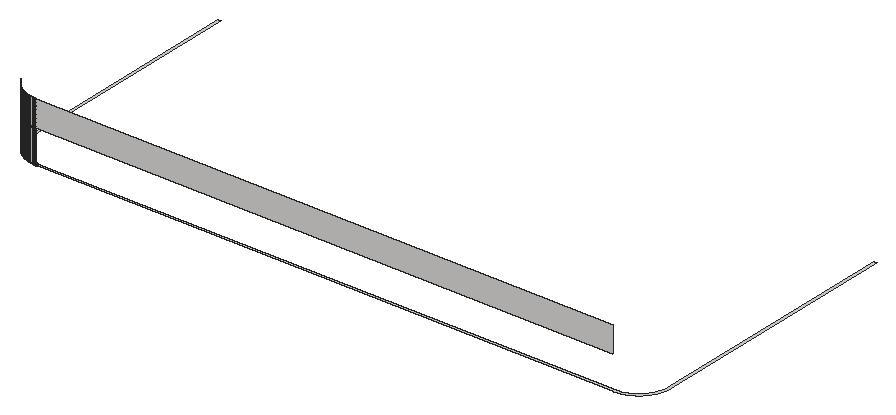
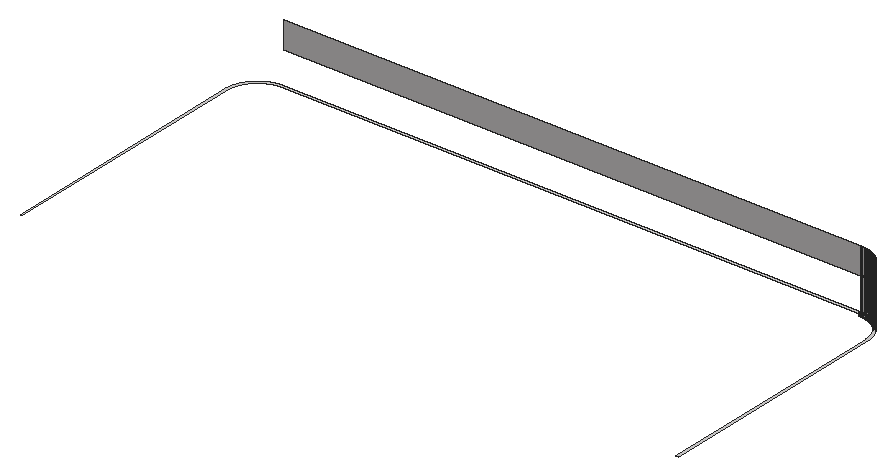
# SketchUp Ruby script. Lengths in inches.
U = 1.inch
M = Sketchup.active_model
def pt(a) = Geom::Point3d.new(a.map { |v| v * U })
def face(e, loops, mat)
  f = e.add_face(loops[0].map { |a| pt(a) })
  loops[1..].each { |l| e.add_face(l.map { |a| pt(a) }).erase! }
  f.material = f.back_material = mat if mat
  f
end
# faces: each face lists its corners as indices into pts; further lists are holes
def faces(e, pts, list, mat = nil) = list.each { |f| face(e, (f[0].is_a?(Array) ? f : [f]).map { |l| l.map { |i| pts[i] } }, mat) }
# xy, xz, yz: faces in a plane at the given z, y or x. An outline is a flat list of corners, or four numbers for a rectangle; further outlines are holes
def ring(l) = l.size == 4 ? [[l[0], l[1]], [l[2], l[1]], [l[2], l[3]], [l[0], l[3]]] : l.each_slice(2).to_a
def flat(e, list, mat, &to3) = list.each { |f| face(e, (f[0].is_a?(Array) ? f : [f]).map { |l| ring(l).map { |u, v| to3.(u, v) } }, mat) }
def xy(e, z, list, mat = nil) = flat(e, list, mat) { |x, y| [x, y, z] }
def xz(e, y, list, mat = nil) = flat(e, list, mat) { |x, z| [x, y, z] }
def yz(e, x, list, mat = nil) = flat(e, list, mat) { |y, z| [x, y, z] }
def lines(e, pts, list) = list.each { |a, b| e.add_line(pt(pts[a]), pt(pts[b])) }
# prism: a flat outline (further loops are holes) pulled along v
def prism(e, loops, v, mat = nil)
  f = face(e, loops, mat); d = Geom::Vector3d.new(v.map { |x| x * U })
  f.pushpull(f.normal.samedirection?(d) ? d.length : -d.length)
end
def box(e, o, s, mat = nil) = prism(e, [[o, [o[0] + s[0], o[1], o[2]], [o[0] + s[0], o[1] + s[1], o[2]], [o[0], o[1] + s[1], o[2]]]], [0, 0, s[2]], mat)
def at(x, y, z, deg = 0) = Geom::Transformation.translation(pt([x, y, z])) * Geom::Transformation.rotation(ORIGIN, Z_AXIS, deg.degrees)
def axes(o, x, y, z) = Geom::Transformation.new([*x, 0, *y, 0, *z, 0, *pt(o).to_a, 1])
def part(name) = M.definitions.add(name)
# library, detail: a bought-in or finely detailed component or shape, given as its bounding box
def library(name, o, s) = part(name).tap { |d| box(d.entities, o, s) }
def detail(e, o, s) = box(e.add_group.entities, o, s)
def put(e, d, t, mat = nil) = e.add_instance(d, t).tap { |i| i.material = mat if mat }
def group(e, t, mat = nil) = e.add_group.tap { |g| g.transformation = t; g.material = mat if mat }.entities
root = M.entities
M.materials.add("[Quartz Light Brown]").color = [215, 212, 212]
xy(root,369,[[215.8,143,215.61,143.01,215.41,143.01,215.21,143.02,215.02,143.03,214.82,143.05,214.63,143.0625,214.43,143.08,214.24,143.1,214.04,143.13,213.85,143.16,213.65,143.18,213.46,143.22,213.27,143.25,213.07,143.29,212.5,143.41,212.12,143.51,211.93,143.5625,211.74,143.62,211.55,143.67,211.36,143.73,211.18,143.8,210.99,143.86,210.81,143.93,210.44,144.07,210.26,144.14,209.54,144.46,209.37,144.55,209.19,144.63,209.02,144.73,208.84,144.82,208.67,144.91,208.16,145.21,208,145.3125,207.83,145.42,207.67,145.53,207.5,145.64,207.18,145.86,207.03,145.98,206.71,146.22,206.56,146.34,206.41,146.47,206.26,146.59,205.96,146.85,205.82,146.99,205.67,147.12,205.53,147.26,205.39,147.39,205.26,147.53,205.12,147.67,204.99,147.82,204.85,147.96,204.59,148.26,204.47,148.41,204.34,148.56,204.22,148.71,203.98,149.03,203.86,149.18,203.64,149.5,203.53,149.67,203.42,149.83,203.3125,150,203.21,150.16,202.91,150.67,202.82,150.84,202.73,151.02,202.63,151.19,202.55,151.37,202.46,151.54,202.14,152.26,202.07,152.44,201.93,152.81,201.86,152.99,201.8,153.18,201.73,153.36,201.67,153.55,201.62,153.74,201.5625,153.93,201.51,154.12,201.41,154.5,201.29,155.07,201.25,155.27,201.22,155.46,201.18,155.65,201.16,155.85,201.13,156.04,201.1,156.24,201.08,156.43,201.0625,156.63,201.05,156.82,201.03,157.02,201.02,157.21,201.01,157.41,201.01,157.61,201,157.8,201,266,202,266,202,157.63,202.02,157.27,202.03,157.08,202.04,156.9,202.08,156.54,202.1,156.35,202.14,155.99,202.23,155.45,202.43,154.55,202.53,154.2,202.58,154.02,202.63,153.85,202.69,153.67,202.74,153.5,202.8,153.33,202.87,153.15,202.93,152.98,203,152.8125,203.07,152.64,203.14,152.47,203.21,152.31,203.29,152.14,203.36,151.97,203.44,151.81,203.53,151.64,203.61,151.48,203.79,151.16,203.875,151,203.97,150.84,204.0625,150.69,204.16,150.53,204.36,150.22,204.46,150.07,204.57,149.92,204.67,149.77,204.89,149.48,205.01,149.33,205.12,149.19,205.24,149.05,205.35,148.91,205.47,148.77,205.6,148.63,205.72,148.5,205.84,148.36,206.36,147.84,206.5,147.72,206.63,147.6,206.77,147.47,206.91,147.35,207.05,147.24,207.19,147.12,207.33,147.01,207.48,146.89,207.77,146.67,207.92,146.57,208.07,146.46,208.22,146.36,208.53,146.16,208.69,146.0625,208.84,145.97,209,145.875,209.16,145.79,209.48,145.61,209.64,145.53,209.81,145.44,209.97,145.36,210.14,145.29,210.31,145.21,210.47,145.14,210.64,145.07,210.8125,145,210.98,144.93,211.15,144.87,211.33,144.8,211.5,144.74,211.67,144.69,211.85,144.63,212.02,144.58,212.2,144.53,212.55,144.43,213.45,144.23,213.99,144.14,214.35,144.1,214.54,144.08,214.9,144.04,215.08,144.03,215.27,144.02,215.63,144,480.37,144,480.73,144.02,480.92,144.03,481.1,144.04,481.46,144.08,481.65,144.1,482.01,144.14,482.55,144.23,483.45,144.43,483.8,144.53,483.98,144.58,484.15,144.63,484.33,144.69,484.5,144.74,484.67,144.8,484.85,144.87,485.02,144.93,485.1875,145,485.36,145.07,485.53,145.14,485.69,145.21,485.86,145.29,486.03,145.36,486.19,145.44,486.36,145.53,486.52,145.61,486.84,145.79,487,145.875,487.16,145.97,487.31,146.0625,487.47,146.16,487.78,146.36,487.93,146.46,488.08,146.57,488.23,146.67,488.52,146.89,488.67,147.01,488.81,147.12,488.95,147.24,489.09,147.35,489.23,147.47,489.37,147.6,489.5,147.72,489.64,147.84,490.16,148.36,490.28,148.5,490.4,148.63,490.53,148.77,490.65,148.91,490.76,149.05,490.88,149.19,490.99,149.33,491.11,149.48,491.33,149.77,491.43,149.92,491.54,150.07,491.64,150.22,491.84,150.53,491.9375,150.69,492.03,150.84,492.125,151,492.21,151.16,492.39,151.48,492.47,151.64,492.56,151.81,492.64,151.97,492.71,152.14,492.79,152.31,492.86,152.47,492.93,152.64,493,152.8125,493.07,152.98,493.13,153.15,493.2,153.33,493.26,153.5,493.31,153.67,493.37,153.85,493.42,154.02,493.47,154.2,493.57,154.55,493.77,155.45,493.86,155.99,493.9,156.35,493.92,156.54,493.96,156.9,493.97,157.08,493.98,157.27,494,157.63,494,275,495,275,495,157.8,494.99,157.61,494.99,157.41,494.98,157.21,494.97,157.02,494.95,156.82,494.9375,156.63,494.92,156.43,494.9,156.24,494.87,156.04,494.84,155.85,494.82,155.65,494.78,155.46,494.75,155.27,494.71,155.07,494.59,154.5,494.49,154.12,494.4375,153.93,494.38,153.74,494.33,153.55,494.27,153.36,494.2,153.18,494.14,152.99,494.07,152.81,493.93,152.44,493.86,152.26,493.54,151.54,493.45,151.37,493.37,151.19,493.27,151.02,493.18,150.84,493.09,150.67,492.79,150.16,492.6875,150,492.58,149.83,492.47,149.67,492.36,149.5,492.14,149.18,492.02,149.03,491.78,148.71,491.66,148.56,491.53,148.41,491.41,148.26,491.15,147.96,491.01,147.82,490.88,147.67,490.74,147.53,490.61,147.39,490.47,147.26,490.33,147.12,490.18,146.99,490.04,146.85,489.74,146.59,489.59,146.47,489.44,146.34,489.29,146.22,488.97,145.98,488.82,145.86,488.5,145.64,488.33,145.53,488.17,145.42,488,145.3125,487.84,145.21,487.33,144.91,487.16,144.82,486.98,144.73,486.81,144.63,486.63,144.55,486.46,144.46,485.74,144.14,485.56,144.07,485.19,143.93,485.01,143.86,484.82,143.8,484.64,143.73,484.45,143.67,484.26,143.62,484.07,143.5625,483.88,143.51,483.5,143.41,482.93,143.29,482.73,143.25,482.54,143.22,482.35,143.18,482.15,143.16,481.96,143.13,481.76,143.1,481.57,143.08,481.37,143.0625,481.18,143.05,480.98,143.03,480.79,143.02,480.59,143.01,480.39,143.01,480.2,143]],"[Quartz Light Brown]")
xz(root,143,[[215.8,369,216,384],[215.8,384,216,396],[216,384,480,396]],"[Quartz Light Brown]")
xz(root,143.01,[[215.41,369,215.61,384],[215.41,384,215.61,396]],"[Quartz Light Brown]")
xz(root,144,[[215.63,368,215.82,369],[215.82,368,216,369]],"[Quartz Light Brown]")
p = [[214.72,144.06,369],[214.72,144.06,368],[214.9,144.04,368],[214.9,144.04,369],[215.08,144.03,368],[215.08,144.03,369],
  [215.27,144.02,368],[215.27,144.02,369],[215.45,144.01,368],[215.45,144.01,369],[215.63,144,368],[215.63,144,369],
  [213.81,144.17,369],[213.81,144.17,368],[213.99,144.14,368],[213.99,144.14,369],[214.17,144.12,368],[214.17,144.12,369],
  [214.35,144.1,368],[214.35,144.1,369],[214.54,144.08,368],[214.54,144.08,369],[213.27,144.27,369],[213.27,144.27,368],
  [213.45,144.23,368],[213.45,144.23,369],[213.63,144.2,368],[213.63,144.2,369],[212.73,144.39,369],[212.73,144.39,368],
  [212.91,144.35,368],[212.91,144.35,369],[213.09,144.31,368],[213.09,144.31,369],[212.375,144.48,369],[212.375,144.48,368],
  [212.55,144.43,368],[212.55,144.43,369],[212.02,144.58,369],[212.02,144.58,368],[212.2,144.53,368],[212.2,144.53,369],
  [211.67,144.69,369],[211.67,144.69,368],[211.85,144.63,368],[211.85,144.63,369],[211.33,144.8,369],[211.33,144.8,368],
  [211.5,144.74,368],[211.5,144.74,369],[211.15,144.87,369],[211.15,144.87,368],[210.8125,145,369],[210.8125,145,368],
  [210.98,144.93,368],[210.98,144.93,369],[210.64,145.07,369],[210.64,145.07,368],[210.31,145.21,369],[210.31,145.21,368],
  [210.47,145.14,368],[210.47,145.14,369],[210.14,145.29,369],[210.14,145.29,368],[209.97,145.36,369],[209.97,145.36,368],
  [209.64,145.53,369],[209.64,145.53,368],[209.81,145.44,368],[209.81,145.44,369],[209.48,145.61,369],[209.48,145.61,368],
  [209.32,145.7,369],[209.32,145.7,368],[209.16,145.79,369],[209.16,145.79,368],[209,145.875,369],[209,145.875,368],
  [208.84,145.97,369],[208.84,145.97,368],[208.69,146.0625,369],[208.69,146.0625,368],[208.53,146.16,369],[208.53,146.16,368],
  [208.375,146.26,369],[208.375,146.26,368],[208.22,146.36,369],[208.22,146.36,368],[208.07,146.46,369],[208.07,146.46,368],
  [207.92,146.57,369],[207.92,146.57,368],[207.77,146.67,369],[207.77,146.67,368],[207.625,146.78,369],[207.625,146.78,368],
  [207.48,146.89,369],[207.48,146.89,368],[207.33,147.01,369],[207.33,147.01,368],[207.19,147.12,369],[207.19,147.12,368],
  [207.05,147.24,369],[207.05,147.24,368],[206.91,147.35,369],[206.91,147.35,368],[206.77,147.47,369],[206.77,147.47,368],
  [206.63,147.6,369],[206.63,147.6,368],[206.5,147.72,369],[206.5,147.72,368],[206.36,147.84,369],[206.36,147.84,368],
  [206.23,147.97,369],[206.23,147.97,368],[206.1,148.1,369],[206.1,148.1,368],[205.97,148.23,369],[205.97,148.23,368],
  [205.84,148.36,369],[205.84,148.36,368],[205.72,148.5,369],[205.72,148.5,368],[205.6,148.63,369],[205.6,148.63,368],
  [205.47,148.77,369],[205.47,148.77,368],[205.35,148.91,369],[205.35,148.91,368],[205.24,149.05,369],[205.24,149.05,368],
  [205.12,149.19,369],[205.12,149.19,368],[205.01,149.33,369],[205.01,149.33,368],[204.89,149.48,369],[204.89,149.48,368],
  [204.78,149.625,369],[204.78,149.625,368],[204.67,149.77,369],[204.67,149.77,368],[204.57,149.92,369],[204.57,149.92,368],
  [204.46,150.07,369],[204.46,150.07,368],[204.36,150.22,369],[204.36,150.22,368],[204.26,150.375,369],[204.26,150.375,368],
  [204.16,150.53,369],[204.16,150.53,368],[204.0625,150.69,369],[204.0625,150.69,368],[203.97,150.84,369],[203.97,150.84,368],
  [203.875,151,369],[203.875,151,368],[214.82,143.05,384],[214.63,143.0625,384],[214.63,143.0625,369],[214.82,143.05,369],
  [215.02,143.03,384],[215.02,143.03,369],[215.21,143.02,384],[215.21,143.02,369],[215.41,143.01,384],[215.41,143.01,369],
  [215.8,143,384],[215.61,143.01,384],[215.61,143.01,369],[215.8,143,369],[214.04,143.13,384],[213.85,143.16,384],
  [213.85,143.16,369],[214.04,143.13,369],[214.24,143.1,384],[214.24,143.1,369],[214.43,143.08,384],[214.43,143.08,369],
  [213.46,143.22,384],[213.27,143.25,384],[213.27,143.25,369],[213.46,143.22,369],[213.65,143.18,384],[213.65,143.18,369],
  [212.88,143.33,384],[212.69,143.37,384],[212.69,143.37,369],[212.88,143.33,369],[213.07,143.29,384],[213.07,143.29,369],
  [212.5,143.41,384],[212.31,143.46,384],[212.31,143.46,369],[212.5,143.41,369],[212.12,143.51,384],[211.93,143.5625,384],
  [211.93,143.5625,369],[212.12,143.51,369],[211.74,143.62,384],[211.55,143.67,384],[211.55,143.67,369],[211.74,143.62,369],
  [211.36,143.73,384],[211.18,143.8,384],[211.18,143.8,369],[211.36,143.73,369],[210.99,143.86,384],[210.99,143.86,369],
  [210.81,143.93,384],[210.625,144,384],[210.625,144,369],[210.81,143.93,369],[210.44,144.07,384],[210.44,144.07,369],
  [210.26,144.14,384],[210.08,144.22,384],[210.08,144.22,369],[210.26,144.14,369],[209.9,144.3,384],[209.9,144.3,369],
  [209.72,144.38,384],[209.72,144.38,369],[209.54,144.46,384],[209.54,144.46,369],[209.37,144.55,384],[209.19,144.63,384],
  [209.19,144.63,369],[209.37,144.55,369],[209.02,144.73,384],[209.02,144.73,369],[208.84,144.82,384],[208.84,144.82,369],
  [208.67,144.91,384],[208.67,144.91,369],[208.5,145.01,384],[208.5,145.01,369],[208.33,145.11,384],[208.33,145.11,369],
  [208.16,145.21,384],[208.16,145.21,369],[208,145.3125,384],[208,145.3125,369],[207.83,145.42,384],[207.83,145.42,369],
  [207.67,145.53,384],[207.67,145.53,369],[207.5,145.64,384],[207.5,145.64,369],[207.34,145.75,384],[207.34,145.75,369],
  [207.18,145.86,384],[207.18,145.86,369],[207.03,145.98,384],[207.03,145.98,369],[206.87,146.1,384],[206.87,146.1,369],
  [206.71,146.22,384],[206.71,146.22,369],[206.56,146.34,384],[206.56,146.34,369],[206.41,146.47,384],[206.41,146.47,369],
  [206.26,146.59,384],[206.26,146.59,369],[206.11,146.72,384],[206.11,146.72,369],[205.96,146.85,384],[205.96,146.85,369],
  [205.82,146.99,384],[205.82,146.99,369],[205.67,147.12,384],[205.67,147.12,369],[205.53,147.26,384],[205.53,147.26,369],
  [205.39,147.39,384],[205.39,147.39,369],[205.26,147.53,384],[205.26,147.53,369],[205.12,147.67,384],[205.12,147.67,369],
  [204.99,147.82,384],[204.99,147.82,369],[204.85,147.96,384],[204.85,147.96,369],[204.72,148.11,384],[204.72,148.11,369],
  [204.59,148.26,384],[204.59,148.26,369],[204.47,148.41,384],[204.47,148.41,369],[204.34,148.56,384],[204.34,148.56,369],
  [204.22,148.71,384],[204.22,148.71,369],[204.1,148.87,384],[204.1,148.87,369],[203.98,149.03,384],[203.98,149.03,369],
  [203.86,149.18,384],[203.86,149.18,369],[203.75,149.34,384],[203.75,149.34,369],[203.64,149.5,384],[203.64,149.5,369],
  [203.53,149.67,384],[203.53,149.67,369],[203.42,149.83,384],[203.42,149.83,369],[203.3125,150,384],[203.3125,150,369],
  [203.21,150.16,384],[203.21,150.16,369],[203.11,150.33,384],[203.11,150.33,369],[203.01,150.5,384],[203.01,150.5,369],
  [202.91,150.67,384],[202.91,150.67,369],[202.82,150.84,384],[202.82,150.84,369],[214.82,143.05,396],[214.63,143.0625,396],
  [214.63,143.0625,384],[214.82,143.05,384],[215.02,143.03,396],[215.02,143.03,384],[215.21,143.02,396],[215.21,143.02,384],
  [215.41,143.01,396],[215.41,143.01,384],[215.8,143,396],[215.61,143.01,396],[215.61,143.01,384],[215.8,143,384],
  [214.04,143.13,396],[213.85,143.16,396],[213.85,143.16,384],[214.04,143.13,384],[214.24,143.1,396],[214.24,143.1,384],
  [214.43,143.08,396],[214.43,143.08,384],[213.46,143.22,396],[213.27,143.25,396],[213.27,143.25,384],[213.46,143.22,384],
  [213.65,143.18,396],[213.65,143.18,384],[212.88,143.33,396],[212.69,143.37,396],[212.69,143.37,384],[212.88,143.33,384],
  [213.07,143.29,396],[213.07,143.29,384],[212.5,143.41,396],[212.31,143.46,396],[212.31,143.46,384],[212.5,143.41,384],
  [212.12,143.51,396],[211.93,143.5625,396],[211.93,143.5625,384],[212.12,143.51,384],[211.74,143.62,396],[211.55,143.67,396],
  [211.55,143.67,384],[211.74,143.62,384],[211.36,143.73,396],[211.18,143.8,396],[211.18,143.8,384],[211.36,143.73,384],
  [210.99,143.86,396],[210.99,143.86,384],[210.81,143.93,396],[210.625,144,396],[210.625,144,384],[210.81,143.93,384],
  [210.44,144.07,396],[210.44,144.07,384],[210.26,144.14,396],[210.08,144.22,396],[210.08,144.22,384],[210.26,144.14,384],
  [209.9,144.3,396],[209.9,144.3,384],[209.72,144.38,396],[209.72,144.38,384],[209.54,144.46,396],[209.54,144.46,384],
  [209.37,144.55,396],[209.19,144.63,396],[209.19,144.63,384],[209.37,144.55,384],[209.02,144.73,396],[209.02,144.73,384],
  [208.84,144.82,396],[208.84,144.82,384],[208.67,144.91,396],[208.67,144.91,384],[208.5,145.01,396],[208.5,145.01,384],
  [208.33,145.11,396],[208.33,145.11,384],[208.16,145.21,396],[208.16,145.21,384],[208,145.3125,396],[208,145.3125,384],
  [207.83,145.42,396],[207.83,145.42,384],[207.67,145.53,396],[207.67,145.53,384],[207.5,145.64,396],[207.5,145.64,384],
  [207.34,145.75,396],[207.34,145.75,384],[207.18,145.86,396],[207.18,145.86,384],[207.03,145.98,396],[207.03,145.98,384],
  [206.87,146.1,396],[206.87,146.1,384],[206.71,146.22,396],[206.71,146.22,384],[206.56,146.34,396],[206.56,146.34,384],
  [206.41,146.47,396],[206.41,146.47,384],[206.26,146.59,396],[206.26,146.59,384],[206.11,146.72,396],[206.11,146.72,384],
  [205.96,146.85,396],[205.96,146.85,384],[205.82,146.99,396],[205.82,146.99,384],[205.67,147.12,396],[205.67,147.12,384],
  [205.53,147.26,396],[205.53,147.26,384],[205.39,147.39,396],[205.39,147.39,384],[205.26,147.53,396],[205.26,147.53,384],
  [205.12,147.67,396],[205.12,147.67,384],[204.99,147.82,396],[204.99,147.82,384],[204.85,147.96,396],[204.85,147.96,384],
  [204.72,148.11,396],[204.72,148.11,384],[204.59,148.26,396],[204.59,148.26,384],[204.47,148.41,396],[204.47,148.41,384],
  [204.34,148.56,396],[204.34,148.56,384],[204.22,148.71,396],[204.22,148.71,384],[204.1,148.87,396],[204.1,148.87,384],
  [203.98,149.03,396],[203.98,149.03,384],[203.86,149.18,396],[203.86,149.18,384],[203.75,149.34,396],[203.75,149.34,384],
  [203.64,149.5,396],[203.64,149.5,384],[203.53,149.67,396],[203.53,149.67,384],[203.42,149.83,396],[203.42,149.83,384],
  [203.3125,150,396],[203.3125,150,384],[203.21,150.16,396],[203.21,150.16,384],[203.11,150.33,396],[203.11,150.33,384],
  [203.01,150.5,396],[203.01,150.5,384],[202.91,150.67,396],[202.91,150.67,384],[202.82,150.84,396],[202.82,150.84,384]]
faces(root,p,[[0,1,2,3],[3,2,4,5],[5,4,6,7],[7,6,8,9],[9,8,10,11],[12,13,14,15],[15,14,16,17],[17,16,18,19],
  [19,18,20,21],[21,20,1,0],[22,23,24,25],[25,24,26,27],[27,26,13,12],[28,29,30,31],[31,30,32,33],[33,32,23,22],
  [34,35,36,37],[37,36,29,28],[38,39,40,41],[41,40,35,34],[42,43,44,45],[45,44,39,38],[46,47,48,49],[49,48,43,42],
  [50,51,47,46],[52,53,54,55],[55,54,51,50],[56,57,53,52],[58,59,60,61],[61,60,57,56],[62,63,59,58],[64,65,63,62],
  [66,67,68,69],[69,68,65,64],[70,71,67,66],[72,73,71,70],[74,75,73,72],[76,77,75,74],[78,79,77,76],[80,81,79,78],
  [82,83,81,80],[84,85,83,82],[86,87,85,84],[88,89,87,86],[90,91,89,88],[92,93,91,90],[94,95,93,92],[96,97,95,94],
  [98,99,97,96],[100,101,99,98],[102,103,101,100],[104,105,103,102],[106,107,105,104],[108,109,107,106],[110,111,109,108],[112,113,111,110],
  [114,115,113,112],[116,117,115,114],[118,119,117,116],[120,121,119,118],[122,123,121,120],[124,125,123,122],[126,127,125,124],[128,129,127,126],
  [130,131,129,128],[132,133,131,130],[134,135,133,132],[136,137,135,134],[138,139,137,136],[140,141,139,138],[142,143,141,140],[144,145,143,142],
  [146,147,145,144],[148,149,147,146],[150,151,149,148],[152,153,151,150],[154,155,153,152],[156,157,155,154],[158,159,160,161],[162,158,161,163],
  [164,162,163,165],[166,164,165,167],[168,169,170,171],[172,173,174,175],[176,172,175,177],[178,176,177,179],[159,178,179,160],[180,181,182,183],
  [184,180,183,185],[173,184,185,174],[186,187,188,189],[190,186,189,191],[181,190,191,182],[192,193,194,195],[187,192,195,188],[196,197,198,199],
  [193,196,199,194],[200,201,202,203],[197,200,203,198],[204,205,206,207],[201,204,207,202],[205,208,209,206],[210,211,212,213],[208,210,213,209],
  [211,214,215,212],[216,217,218,219],[214,216,219,215],[217,220,221,218],[220,222,223,221],[222,224,225,223],[226,227,228,229],[224,226,229,225],
  [227,230,231,228],[230,232,233,231],[232,234,235,233],[234,236,237,235],[236,238,239,237],[238,240,241,239],[240,242,243,241],[242,244,245,243],
  [244,246,247,245],[246,248,249,247],[248,250,251,249],[250,252,253,251],[252,254,255,253],[254,256,257,255],[256,258,259,257],[258,260,261,259],
  [260,262,263,261],[262,264,265,263],[264,266,267,265],[266,268,269,267],[268,270,271,269],[270,272,273,271],[272,274,275,273],[274,276,277,275],
  [276,278,279,277],[278,280,281,279],[280,282,283,281],[282,284,285,283],[284,286,287,285],[286,288,289,287],[288,290,291,289],[290,292,293,291],
  [292,294,295,293],[294,296,297,295],[296,298,299,297],[298,300,301,299],[300,302,303,301],[302,304,305,303],[304,306,307,305],[306,308,309,307],
  [308,310,311,309],[310,312,313,311],[312,314,315,313],[314,316,317,315],[316,318,319,317],[318,320,321,319],[322,323,324,325],[326,322,325,327],
  [328,326,327,329],[330,328,329,331],[332,333,334,335],[336,337,338,339],[340,336,339,341],[342,340,341,343],[323,342,343,324],[344,345,346,347],
  [348,344,347,349],[337,348,349,338],[350,351,352,353],[354,350,353,355],[345,354,355,346],[356,357,358,359],[351,356,359,352],[360,361,362,363],
  [357,360,363,358],[364,365,366,367],[361,364,367,362],[368,369,370,371],[365,368,371,366],[369,372,373,370],[374,375,376,377],[372,374,377,373],
  [375,378,379,376],[380,381,382,383],[378,380,383,379],[381,384,385,382],[384,386,387,385],[386,388,389,387],[390,391,392,393],[388,390,393,389],
  [391,394,395,392],[394,396,397,395],[396,398,399,397],[398,400,401,399],[400,402,403,401],[402,404,405,403],[404,406,407,405],[406,408,409,407],
  [408,410,411,409],[410,412,413,411],[412,414,415,413],[414,416,417,415],[416,418,419,417],[418,420,421,419],[420,422,423,421],[422,424,425,423],
  [424,426,427,425],[426,428,429,427],[428,430,431,429],[430,432,433,431],[432,434,435,433],[434,436,437,435],[436,438,439,437],[438,440,441,439],
  [440,442,443,441],[442,444,445,443],[444,446,447,445],[446,448,449,447],[448,450,451,449],[450,452,453,451],[452,454,455,453],[454,456,457,455],
  [456,458,459,457],[458,460,461,459],[460,462,463,461],[462,464,465,463],[464,466,467,465],[466,468,469,467],[468,470,471,469],[470,472,473,471],
  [472,474,475,473],[474,476,477,475],[476,478,479,477],[478,480,481,479],[480,482,483,481],[482,484,485,483]],"[Quartz Light Brown]")
